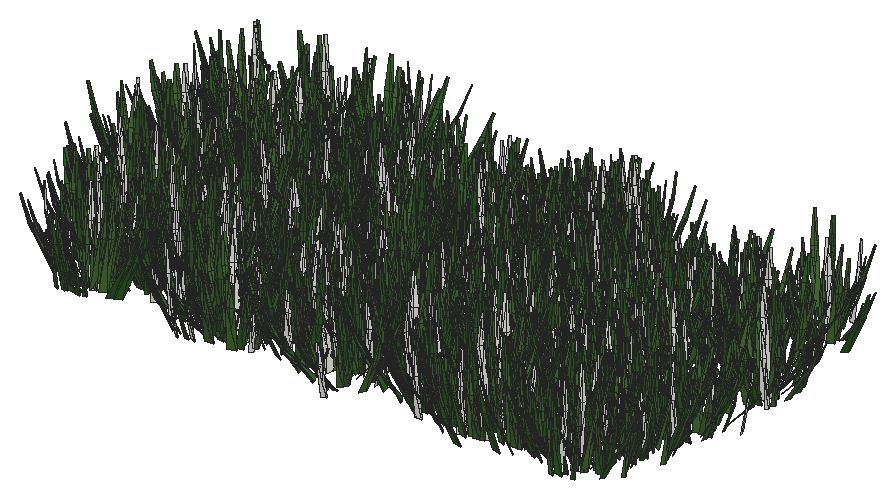
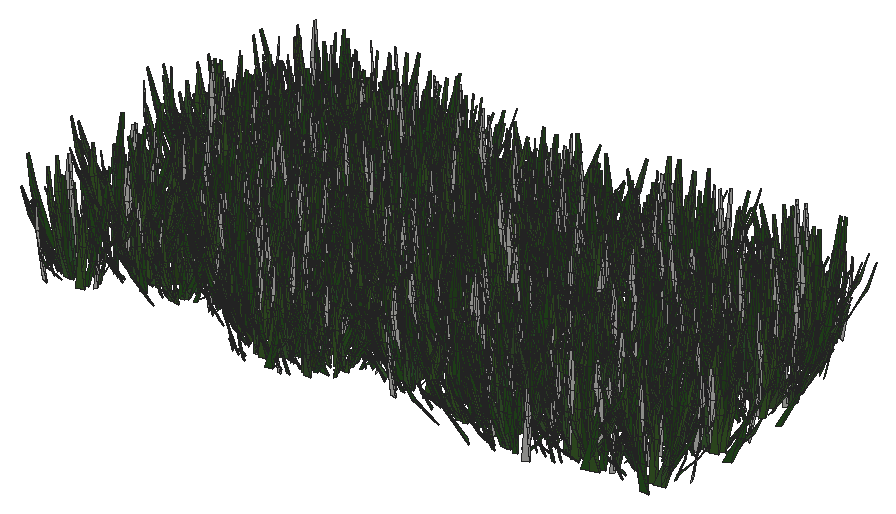
# SketchUp Ruby script. Lengths in inches.
U = 1.inch
M = Sketchup.active_model
def pt(a) = Geom::Point3d.new(a.map { |v| v * U })
def face(e, loops, mat)
  f = e.add_face(loops[0].map { |a| pt(a) })
  loops[1..].each { |l| e.add_face(l.map { |a| pt(a) }).erase! }
  f.material = f.back_material = mat if mat
  f
end
# faces: each face lists its corners as indices into pts; further lists are holes
def faces(e, pts, list, mat = nil) = list.each { |f| face(e, (f[0].is_a?(Array) ? f : [f]).map { |l| l.map { |i| pts[i] } }, mat) }
# xy, xz, yz: faces in a plane at the given z, y or x. An outline is a flat list of corners, or four numbers for a rectangle; further outlines are holes
def ring(l) = l.size == 4 ? [[l[0], l[1]], [l[2], l[1]], [l[2], l[3]], [l[0], l[3]]] : l.each_slice(2).to_a
def flat(e, list, mat, &to3) = list.each { |f| face(e, (f[0].is_a?(Array) ? f : [f]).map { |l| ring(l).map { |u, v| to3.(u, v) } }, mat) }
def xy(e, z, list, mat = nil) = flat(e, list, mat) { |x, y| [x, y, z] }
def xz(e, y, list, mat = nil) = flat(e, list, mat) { |x, z| [x, y, z] }
def yz(e, x, list, mat = nil) = flat(e, list, mat) { |y, z| [x, y, z] }
def lines(e, pts, list) = list.each { |a, b| e.add_line(pt(pts[a]), pt(pts[b])) }
# prism: a flat outline (further loops are holes) pulled along v
def prism(e, loops, v, mat = nil)
  f = face(e, loops, mat); d = Geom::Vector3d.new(v.map { |x| x * U })
  f.pushpull(f.normal.samedirection?(d) ? d.length : -d.length)
end
def box(e, o, s, mat = nil) = prism(e, [[o, [o[0] + s[0], o[1], o[2]], [o[0] + s[0], o[1] + s[1], o[2]], [o[0], o[1] + s[1], o[2]]]], [0, 0, s[2]], mat)
def at(x, y, z, deg = 0) = Geom::Transformation.translation(pt([x, y, z])) * Geom::Transformation.rotation(ORIGIN, Z_AXIS, deg.degrees)
def axes(o, x, y, z) = Geom::Transformation.new([*x, 0, *y, 0, *z, 0, *pt(o).to_a, 1])
def part(name) = M.definitions.add(name)
# library, detail: a bought-in or finely detailed component or shape, given as its bounding box
def library(name, o, s) = part(name).tap { |d| box(d.entities, o, s) }
def detail(e, o, s) = box(e.add_group.entities, o, s)
def put(e, d, t, mat = nil) = e.add_instance(d, t).tap { |i| i.material = mat if mat }
def group(e, t, mat = nil) = e.add_group.tap { |g| g.transformation = t; g.material = mat if mat }.entities
root = M.entities
M.materials.add("Material1").color = [58, 110, 58]
M.materials.add("Material10").color = [48, 100, 38]
M.materials.add("Material3").color = [68, 110, 58]
M.materials.add("Material4").color = [48, 90, 38]
M.materials.add("Material5").color = [68, 110, 48]
M.materials.add("Material6").color = [48, 90, 48]
M.materials.add("Material8").color = [58, 90, 38]
M.materials.add("Material9").color = [68, 100, 58]
c1 = part("grass00")
p = [[-0.6875,0.15,0],[-0.56,0.08,5.52],[-0.04,0.03,2.76],[0.48,-0.02,0],[0.35,-0.02,5.52],[-0.1,-0.14,5.52],
  [-0.12,0.65,8.37],[-0.42,0.65,8.37]]
faces(c1.entities,p,[[0,1,2,3],[3,2,4],[1,5,2],[5,4,2],[1,6,5],[4,5,6],[7,6,1]])
c2 = part("Group16\#1")
put(c2.entities,c1,axes([1.44,-0.61,-0.01],[0.05352,0.12609,0],[-0.10704,0.04543,0.07239],[0.06664,-0.02828,0.11628]),"Material6")
put(c2.entities,c1,axes([0.76,-0.15,-0.01],[0.04676,0.24062,0],[-0.23162,0.04501,0.06642],[0.0652,-0.01267,0.23595]),"Material3")
put(c2.entities,c1,axes([0.79,0.01,-0.01],[-0.00606,0.34651,0],[-0.34381,-0.00602,0.0432],[0.04319,0.00076,0.34386]))
put(c2.entities,c1,axes([1,0.23,-0.01],[-0.07192,0.31144,0],[-0.28722,-0.06632,0.1236],[0.12043,0.02781,0.29478]),"Material5")
put(c2.entities,c1,axes([1.66,0.77,-0.01],[-0.13828,0.29651,0],[-0.21551,-0.1005,0.22471],[0.20365,0.09498,0.23779]),"Material10")
put(c2.entities,c1,axes([0.6875,0.52,-0.01],[-0.18126,0.24051,0],[-0.22746,-0.17142,0.09788],[0.07817,0.05891,0.28481]),"Material5")
put(c2.entities,c1,axes([0.68,0.78,-0.01],[-0.215,0.18688,0],[-0.12385,-0.14248,0.21334],[0.13995,0.16101,0.18878]),"Material3")
put(c2.entities,c1,axes([0.56,1,-0.01],[-0.13756,0.07624,0],[-0.06159,-0.11112,0.0927],[0.04494,0.08108,0.12705]),"Material5")
put(c2.entities,c1,axes([0.2,0.64,-0.01],[-0.23729,0.07254,0],[-0.05711,-0.18681,0.153],[0.04473,0.14632,0.19535]),"Material10")
put(c2.entities,c1,axes([0.0625,0.72,-0.01],[-0.28874,0.02525,0],[-0.02179,-0.24916,0.14647],[0.01276,0.14591,0.25012]),"Material3")
put(c2.entities,c1,axes([-0.08,0.62,-0.01],[-0.34089,-0.04187,0],[0.03255,-0.26504,0.216],[-0.02633,0.21439,0.26703]),"Material10")
put(c2.entities,c1,axes([-0.34,0.98,-0.01],[-0.14314,-0.0493,0],[0.04397,-0.12769,0.06843],[-0.02228,0.0647,0.13505]),"Material10")
put(c2.entities,c1,axes([-0.87,1.45,-0.01],[-0.23488,-0.14114,0],[0.13761,-0.22901,0.06087],[-0.03135,0.05217,0.26717]))
put(c2.entities,c1,axes([-0.72,0.77,-0.01],[-0.14208,-0.13251,0],[0.07209,-0.0773,0.16301],[-0.11118,0.11922,0.1057]),"Material10")
put(c2.entities,c1,axes([-0.62,0.43,-0.01],[-0.14845,-0.21203,0],[0.18654,-0.13061,0.12304],[-0.10079,0.07057,0.22772]),"Material3")
put(c2.entities,c1,axes([-0.68,0.29,-0.01],[-0.13639,-0.32136,0],[0.31723,-0.13464,0.05579],[-0.05136,0.0218,0.34462]),"Material4")
put(c2.entities,c1,axes([-0.64,0.125,-0.01],[-0.0458,-0.23569,0],[0.22124,-0.043,0.08276],[-0.08124,0.01579,0.22538]),"Material1")
put(c2.entities,c1,axes([-1.6,-0.03,-0.01],[0.00576,-0.32897,0],[0.27526,0.00482,0.18018],[-0.18015,-0.00315,0.2753]),"Material5")
put(c2.entities,c1,axes([-1.36,-0.31,-0.01],[0.05718,-0.24765,0],[0.18172,0.04196,0.17267],[-0.16825,-0.03885,0.1865]),"Material10")
put(c2.entities,c1,axes([-1.54,-0.72,-0.01],[0.06537,-0.14017,0],[0.13555,0.06321,0.03939],[-0.0357,-0.01665,0.14956]))
put(c2.entities,c1,axes([-1.19,-0.9,-0.01],[0.09597,-0.12735,0],[0.11214,0.08451,0.07557],[-0.06035,-0.04548,0.14042]),"Material9")
put(c2.entities,c1,axes([-0.47,-0.54,-0.01],[0.11588,-0.10072,0],[0.0618,0.0711,0.12124],[-0.07953,-0.0915,0.0942]))
put(c2.entities,c1,axes([-0.47,-0.84,-0.01],[0.11927,-0.0661,0],[0.06603,0.11913,0.00646],[-0.00313,-0.00565,0.13621]),"Material5")
put(c2.entities,c1,axes([-0.38,-1.24,-0.01],[0.28037,-0.08571,0],[0.0618,0.20215,0.20315],[-0.05939,-0.19428,0.21139]),"Material9")
put(c2.entities,c1,axes([-0.06,-0.66,-0.01],[0.22719,-0.01987,0],[0.01247,0.14255,0.17758],[-0.01547,-0.17691,0.1431]),"Material8")
put(c2.entities,c1,axes([0.11,-0.89,-0.01],[0.14882,0.01828,0],[-0.01058,0.08611,0.12229],[0.01491,-0.12138,0.08676]),"Material6")
put(c2.entities,c1,axes([0.25,-0.72,-0.01],[0.20481,0.07053,0],[-0.06206,0.18022,0.10291],[0.03351,-0.0973,0.1906]),"Material6")
put(c2.entities,c1,axes([0.85,-1.42,-0.01],[0.16481,0.09904,0],[-0.09472,0.15762,0.05616],[0.02893,-0.04814,0.18389]),"Material5")
put(c2.entities,c1,axes([1.01,-1.09,-0.01],[0.21858,0.20385,0],[-0.17495,0.1876,0.15339],[0.10462,-0.11218,0.25652]),"Material10")
put(c2.entities,c1,axes([1.01,-0.71,-0.01],[0.08733,0.12473,0],[-0.06445,0.04512,0.13037],[0.1068,-0.07477,0.07867]),"Material6")
c3 = part("Group15\#1")
put(c3.entities,c2,at(0,0,0))
c4 = part("3darcstudiotree_grass00\#1")
put(c4.entities,c3,at(0,0,0))
put(root,c4,axes([299.78,141.87,0.25],[-0.51577,0.72337,0],[-1.03322,-0.50751,-0.04665],[-0.04944,-0.02429,1.47851]))
put(root,c4,axes([300.08,145.62,0.25],[0.04993,0.88338,0],[-1.12828,0.04393,-0.04808],[-0.07252,0.00282,1.70557]))
put(root,c4,axes([300.54,138.19,0.25],[-1.00125,0.60358,0],[-0.57545,-0.65762,-0.02785],[-0.03086,-0.03527,1.84622]))
put(root,c4,axes([300.73,137.15,0.25],[-0.28415,-0.883,0],[1.03818,-0.23015,-0.04991],[0.05947,-0.01318,1.32514]))
put(root,c4,axes([300.77,136.11,0.25],[0.54173,-0.92093,0],[0.98628,0.39968,-0.03421],[0.05303,0.02149,1.89316]))
put(root,c4,axes([301.14,134.74,0.25],[-0.01613,-0.76479,0],[1.13568,-0.0165,-0.04239],[0.05311,-0.00077,1.42343]))
put(root,c4,axes([301.49,140.1,0.25],[-0.02649,0.7502,0],[-0.93326,-0.0227,-0.04664],[-0.07074,-0.00172,1.41669]))
put(root,c4,axes([301.48,142.71,0.25],[0.76423,0.72762,0],[-0.68872,0.49833,-0.0286],[-0.04274,0.03093,1.81122]))
put(root,c4,axes([302.39,132.09,0.25],[-0.43129,0.73346,0],[-1.07574,-0.43577,-0.02753],[-0.03805,-0.01541,1.84121]))
put(root,c4,axes([302.49,133.8,0.25],[0.56343,-0.63153,0],[0.788,0.48432,-0.04843],[0.0685,0.0421,1.72564]))
put(root,c4,axes([303.03,137.14,0.25],[0.05508,-0.79039,0],[1.0526,0.05053,-0.03098],[0.04607,0.00221,1.57088]))
put(root,c4,axes([303.125,136.4375,0.25],[-0.10182,-0.84072,0],[1.03842,-0.08664,-0.02999],[0.05463,-0.00456,1.91089]))
put(root,c4,axes([303.05,145.8,0.25],[0.5504,-0.80783,0],[1.00535,0.47188,-0.04614],[0.05165,0.02424,1.48544]))
put(root,c4,axes([303.06,130.6,0.25],[0.88072,-0.75596,0],[0.79178,0.63548,-0.03201],[0.03942,0.03164,1.88682]))
put(root,c4,axes([303.72,130.48,0.25],[0.67514,-0.58996,0],[0.84636,0.66723,-0.03691],[0.04374,0.03448,1.90749]))
put(root,c4,axes([304.05,135.15,0.25],[-0.82491,-0.8058,0],[0.91289,-0.64381,-0.06095],[0.06828,-0.04816,1.76096]))
put(root,c4,axes([304.2,140.98,0.25],[-1.06648,-0.29234,0],[0.33481,-0.84142,-0.04962],[0.02631,-0.06612,1.8049]))
put(root,c4,axes([304.03,136.32,0.25],[-0.77838,0.37748,0],[-0.59922,-0.85123,-0.05376],[-0.03154,-0.04481,1.38154]))
put(root,c4,axes([303.89,142.53,0.25],[-0.25153,0.98585,0],[-1.19968,-0.21086,-0.05285],[-0.07259,-0.01276,1.72177]))
put(root,c4,axes([304.6,139.4,0.25],[-1.0477,-0.13596,0],[0.1947,-1.03362,-0.04342],[0.00888,-0.04717,1.66984]))
put(root,c4,axes([304.31,145.87,0.25],[-0.53647,0.96882,0],[-1.0534,-0.40184,-0.02861],[-0.04227,-0.01613,1.88512]))
put(root,c4,axes([304.62,138.11,0.25],[-0.94495,-0.04978,0],[0.07876,-1.02991,-0.04372],[0.00292,-0.03822,1.31241]))
put(root,c4,axes([304.66,133.875,0.25],[0.88611,-0.32919,0],[0.4327,0.80239,-0.04939],[0.03441,0.06381,1.80606]))
put(root,c4,axes([305.41,132.12,0.25],[-0.97721,-0.2509,0],[0.37297,-1.00075,-0.06046],[0.02106,-0.05652,1.48798]))
put(root,c4,axes([306.02,142.74,0.25],[1.14716,0.41931,0],[-0.39995,0.75378,-0.04159],[-0.02402,0.04527,1.42181]))
put(root,c4,axes([306.17,139.4375,0.25],[0.27344,1.00751,0],[-1.06134,0.19844,-0.04632],[-0.06652,0.01244,1.6013]))
put(root,c4,axes([307.21,143.59,0.25],[-0.92535,-0.73173,0],[0.88977,-0.77516,-0.03405],[0.02665,-0.02322,1.46358]))
put(root,c4,axes([306.67,138.9,0.25],[0.38479,0.87258,0],[-1.09891,0.33384,-0.03042],[-0.03924,0.01192,1.60735]))
put(root,c4,axes([306.79,147.18,0.25],[1.0966,0.3645,0],[-0.41445,0.85898,-0.05201],[-0.03051,0.06323,1.75905]))
put(root,c4,axes([307.11,134.75,0.25],[-0.02724,0.8884,0],[-1.06639,-0.02253,-0.03168],[-0.04928,-0.00104,1.66016]))
put(root,c4,axes([307.14,142.44,0.25],[0.47063,0.99955,0],[-1.01276,0.3285,-0.05423],[-0.06364,0.02064,1.37014]))
put(root,c4,axes([307.41,133.73,0.25],[-0.66435,0.90789,0],[-1.02818,-0.5183,-0.06137],[-0.06369,-0.03211,1.46064]))
put(root,c4,axes([307.32,136.98,0.25],[0.98353,-0.2674,0],[0.31916,0.80872,-0.03684],[0.0181,0.04586,1.61813]))
put(root,c4,axes([307.6,145.88,0.25],[0.72927,0.8559,0],[-0.97666,0.57329,-0.03132],[-0.03828,0.02247,1.7905]))
put(root,c4,axes([308.45,141.2,0.25],[-0.57612,-0.75798,0],[0.99797,-0.52255,-0.04882],[0.04842,-0.02535,1.38366]))
put(root,c4,axes([308.22,138.1,0.25],[1.07822,-0.4599,0],[0.58685,0.94782,-0.04443],[0.02209,0.03568,1.39643]))
put(root,c4,axes([308.5625,143.11,0.25],[-0.5579,-0.63099,0],[1.01432,-0.61782,-0.05528],[0.06314,-0.03846,1.78248]))
put(root,c4,axes([308.57,142.55,0.25],[-1.00665,-0.38225,0],[0.39719,-0.72058,-0.02741],[0.0223,-0.04045,1.86713]))
put(root,c4,axes([308.5625,131.11,0.25],[-0.96516,0.38443,0],[-0.43122,-0.74583,-0.02803],[-0.02343,-0.04053,1.92571]))
put(root,c4,axes([308.45,139.83,0.25],[1.05725,-0.32469,0],[0.33364,0.74841,-0.04569],[0.02936,0.06585,1.78027]))
put(root,c4,axes([308.57,133.29,0.25],[1.21894,-0.05836,0],[0.05945,0.85542,-0.03809],[0.00382,0.05491,1.79573]))
put(root,c4,axes([308.69,132.48,0.25],[1.08674,-0.51423,0],[0.5096,0.74191,-0.05304],[0.04758,0.06927,1.86337]))
put(root,c4,axes([309.62,144.6875,0.25],[0.96211,-0.31155,0],[0.3285,0.69886,-0.03886],[0.02375,0.05053,1.52001]))
put(root,c4,axes([309.84,133.23,0.25],[0.18176,0.81903,0],[-1.09456,0.16733,-0.0472],[-0.06112,0.00934,1.46547]))
put(root,c4,axes([309.86,146.21,0.25],[0.71429,0.86085,0],[-0.78996,0.45156,-0.04649],[-0.05198,0.02971,1.30192]))
put(root,c4,axes([309.89,139.42,0.25],[1.04874,0.16215,0],[-0.17266,0.76932,-0.03922],[-0.01113,0.04958,1.46066]))
put(root,c4,axes([310.47,137,0.25],[-0.34398,-0.78173,0],[0.86639,-0.26263,-0.03784],[0.06395,-0.01938,1.65933]))
put(root,c4,axes([310.63,141.27,0.25],[1.04153,-0.54846,0],[0.60752,0.79477,-0.04672],[0.04077,0.05334,1.84728]))
put(root,c4,axes([310.46,130.5625,0.25],[0.92621,0.73809,0],[-0.85701,0.74087,-0.04664],[-0.04646,0.04016,1.77978]))
put(root,c4,axes([311.28,143.21,0.25],[0.57087,-0.64299,0],[0.86179,0.52709,-0.04551],[0.05625,0.0344,1.64335]))
put(root,c4,axes([311.53,130.5625,0.25],[-0.46204,0.65988,0],[-1.12301,-0.5417,-0.02835],[-0.03266,-0.01575,1.73088]))
put(root,c4,axes([312.01,144.46,0.25],[-1.01342,0.10573,0],[-0.15227,-1.00541,-0.04842],[-0.00964,-0.06363,1.94818]))
put(root,c4,axes([311.79,142.55,0.25],[1.26054,0.10801,0],[-0.1304,1.04837,-0.06196],[-0.00771,0.06201,1.53928]))
put(root,c4,axes([311.85,134.45,0.25],[1.00305,0.14539,0],[-0.20705,0.98408,-0.04039],[-0.00807,0.03835,1.39779]))
put(root,c4,axes([311.91,141.29,0.25],[0.92598,0.55829,0],[-0.67255,0.76846,-0.05492],[-0.04623,0.05283,1.63919]))
put(root,c4,axes([312.95,132.18,0.25],[-1.15018,-0.15887,0],[0.16599,-0.8279,-0.03971],[0.00952,-0.04747,1.4765]))
put(root,c4,axes([312.78,136.05,0.25],[0.82997,-0.75391,0],[0.73924,0.56064,-0.04297],[0.04689,0.03556,1.48019]))
put(root,c4,axes([313.24,141.47,0.25],[0.34968,-0.96719,0],[0.98733,0.24591,-0.0465],[0.06293,0.01567,1.45674]))
put(root,c4,axes([312.98,134.48,0.25],[1.12096,-0.03668,0],[0.04224,0.88921,-0.03451],[0.00237,0.04996,1.8714]))
put(root,c4,axes([312.97,133.34,0.25],[0.94146,0.27887,0],[-0.40298,0.93723,-0.03925],[-0.0143,0.03327,1.29995]))
put(root,c4,axes([313.625,139.54,0.25],[-0.01858,-0.90757,0],[1.28861,-0.01817,-0.0635],[0.09505,-0.00134,1.92948]))
put(root,c4,axes([313.75,145.91,0.25],[0.98461,-0.38374,0],[0.39191,0.69275,-0.03796],[0.02677,0.04732,1.52986]))
put(root,c4,axes([314.42,143.93,0.25],[-0.34623,-0.72321,0],[1.04472,-0.34455,-0.04918],[0.05465,-0.01802,1.34418]))
put(root,c4,axes([314.54,145.03,0.25],[0.15043,-0.7527,0],[1.21044,0.16665,-0.06063],[0.07503,0.01033,1.53907]))
put(root,c4,axes([314.73,138.17,0.25],[0.39909,-0.81566,0],[1.02034,0.34393,-0.04502],[0.07048,0.02376,1.86083]))
put(root,c4,axes([314.98,133.11,0.25],[-0.27504,-0.89282,0],[1.07963,-0.22912,-0.04783],[0.06688,-0.01419,1.6084]))
put(root,c4,axes([314.77,131.41,0.25],[1.24297,0.07238,0],[-0.08345,0.98727,-0.05051],[-0.00566,0.06702,1.91076]))
put(root,c4,axes([315.16,136.78,0.25],[0.44545,-0.68346,0],[1.06425,0.47785,-0.03985],[0.0435,0.01953,1.5017]))
put(root,c4,axes([315.03,142.12,0.25],[1.14321,0.40608,0],[-0.51013,0.98935,-0.06274],[-0.03659,0.07096,1.92197]))
put(root,c4,axes([315.69,137.68,0.25],[-1.0413,-0.45924,0],[0.51605,-0.8061,-0.03648],[0.0279,-0.04359,1.79293]))
put(root,c4,axes([316.17,132.56,0.25],[0.8304,0.29143,0],[-0.37726,0.74054,-0.04149],[-0.03179,0.0624,1.90578]))
put(root,c4,axes([316.15,133.21,0.25],[1.10631,0.33098,0],[-0.3979,0.91621,-0.05978],[-0.02583,0.05947,1.49495]))
put(root,c4,axes([316.4375,134.86,0.25],[0.42473,-0.75301,0],[0.8196,0.31847,-0.04141],[0.08184,0.0318,1.97468]))
put(root,c4,axes([316.54,141.47,0.25],[-0.21123,0.7691,0],[-0.89914,-0.17012,-0.03421],[-0.06786,-0.01284,1.87625]))
put(root,c4,axes([317.21,133.19,0.25],[-1.12613,-0.03411,0],[0.04109,-0.93447,-0.04384],[0.00237,-0.05387,1.66887]))
put(root,c4,axes([317.4375,131.97,0.25],[-0.97309,0.51402,0],[-0.49262,-0.64245,-0.04609],[-0.04607,-0.06009,1.7083]))
put(root,c4,axes([317.63,134.71,0.25],[-0.64125,-0.58627,0],[0.90023,-0.67833,-0.05879],[0.05947,-0.04481,1.66118]))
put(root,c4,axes([317.62,130.52,0.25],[-0.97091,0.18786,0],[-0.29032,-1.03362,-0.06463],[-0.01526,-0.05435,1.33032]))
put(root,c4,axes([317.6875,142.18,0.25],[-0.0786,-0.93173,0],[1.13363,-0.06588,-0.04142],[0.06279,-0.00365,1.72685]))
put(root,c4,axes([317.33,146.08,0.25],[0.35004,0.7486,0],[-1.10063,0.35454,-0.04732],[-0.05301,0.01708,1.41896]))
put(root,c4,axes([317.71,140.87,0.25],[1.16212,0.12281,0],[-0.11865,0.77346,-0.04636],[-0.01154,0.07525,1.85211]))
put(root,c4,axes([318.25,147.34,0.25],[-0.69384,-0.6726,0],[0.85793,-0.60969,-0.03189],[0.03287,-0.02336,1.53238]))
put(root,c4,axes([318.26,138.55,0.25],[0.89894,0.06975,0],[-0.1065,0.94557,-0.04931],[-0.00617,0.05478,1.538]))
put(root,c4,axes([318.9,142.34,0.25],[0.3076,0.88313,0],[-0.9496,0.22786,-0.04889],[-0.06973,0.01673,1.46761]))
put(root,c4,axes([319.32,133.625,0.25],[0.44989,-0.65828,0],[1.12235,0.52842,-0.03953],[0.04723,0.02224,1.77239]))
put(root,c4,axes([319.52,138.32,0.25],[-0.95818,-0.32844,0],[0.39605,-0.79597,-0.04671],[0.03185,-0.06401,1.85324]))
put(root,c4,axes([319.27,134.52,0.25],[0.25037,1.00901,0],[-1.01055,0.17274,-0.03105],[-0.05539,0.00947,1.87912]))
put(root,c4,axes([319.34,137.24,0.25],[0.35055,1.00246,0],[-0.90433,0.21786,-0.03743],[-0.0536,0.01291,1.40382]))
put(root,c4,axes([319.48,143.4,0.25],[0.66113,0.53342,0],[-0.84049,0.71763,-0.04673],[-0.03929,0.03355,1.45453]))
put(root,c4,axes([319.6,144.55,0.25],[1.17347,-0.27786,0],[0.3552,1.03341,-0.04256],[0.01402,0.0408,1.55488]))
put(root,c4,axes([319.69,145.62,0.25],[0.1752,0.94217,0],[-0.95925,0.12288,-0.04631],[-0.07803,0.01,1.65491]))
put(root,c4,axes([319.8125,146.87,0.25],[0.28963,0.74847,0],[-0.93547,0.24938,-0.04361],[-0.06802,0.01813,1.60948]))
put(root,c4,axes([320.26,139.86,0.25],[-0.06585,-0.80008,0],[1.09119,-0.06187,-0.04502],[0.05343,-0.00303,1.30109]))
put(root,c4,axes([320.76,147.34,0.25],[-0.46015,0.96018,0],[-0.861,-0.28426,-0.04072],[-0.06272,-0.02071,1.53595]))
put(root,c4,axes([320.88,141.8,0.25],[1.02393,-0.20893,0],[0.23736,0.80136,-0.02888],[0.01203,0.04061,1.73467]))
put(root,c4,axes([321.84,131.28,0.25],[-1.12621,0.19113,0],[-0.2015,-0.81791,-0.0347],[-0.01115,-0.04525,1.61275]))
put(root,c4,axes([322.08,140.71,0.25],[0.06137,-0.83271,0],[1.13269,0.05751,-0.05271],[0.06386,0.00324,1.37729]))
put(root,c4,axes([322.02,131.74,0.25],[0.54931,-0.6716,0],[0.75634,0.42617,-0.03969],[0.0509,0.02868,1.41714]))
put(root,c4,axes([322.27,138.85,0.25],[-0.78066,-0.67204,0],[0.68687,-0.54967,-0.03577],[0.04031,-0.03226,1.49339]))
put(root,c4,axes([321.93,137.24,0.25],[0.27982,0.75631,0],[-1.1229,0.28621,-0.03259],[-0.04697,0.01197,1.77089]))
put(root,c4,axes([321.93,145.23,0.25],[0.80316,0.707,0],[-0.70311,0.55026,-0.02839],[-0.0403,0.03154,1.88589]))
put(root,c4,axes([322.77,145.93,0.25],[-1.10827,0.13604,0],[-0.16547,-0.92861,-0.04443],[-0.01051,-0.05896,1.82802]))
put(root,c4,axes([323.32,142.65,0.25],[-0.86841,-0.52371,0],[0.68358,-0.78087,-0.03763],[0.03701,-0.04227,1.94544]))
put(root,c4,axes([323.41,137.35,0.25],[-0.91874,-0.68883,0],[0.79509,-0.73056,-0.0585],[0.0631,-0.05798,1.90866]))
put(root,c4,axes([323.25,141.46,0.25],[-0.34506,0.75478,0],[-0.92362,-0.29088,-0.03389],[-0.05306,-0.01671,1.65454]))
put(root,c4,axes([323.57,131.22,0.25],[-0.92977,-0.22168,0],[0.33206,-0.95946,-0.05258],[0.02224,-0.06426,1.84274]))
put(root,c4,axes([323.69,135.52,0.25],[-0.02074,-0.84875,0],[1.20005,-0.0202,-0.05384],[0.05935,-0.001,1.32332]))
put(root,c4,axes([323.71,145.12,0.25],[-1.03502,0.33572,0],[-0.32811,-0.69686,-0.02866],[-0.02179,-0.04627,1.88291]))
put(root,c4,axes([323.92,140.11,0.25],[-0.92041,-0.50708,0],[0.71428,-0.89316,-0.03911],[0.02409,-0.03012,1.43856]))
put(root,c4,axes([323.76,134.42,0.25],[-0.00089,-0.79123,0],[0.93063,-0.00072,-0.0371],[0.07359,-0.00006,1.84609]))
put(root,c4,axes([323.72,133.85,0.25],[0.98992,-0.58841,0],[0.73097,0.84717,-0.04389],[0.03917,0.04539,1.92393]))
put(root,c4,axes([324.01,132.55,0.25],[1.03159,-0.24301,0],[0.31461,0.92006,-0.03157],[0.01327,0.0388,1.77323]))
put(root,c4,axes([324.93,137.42,0.25],[-0.37538,-0.75879,0],[1.02359,-0.34885,-0.04381],[0.0639,-0.02178,1.74465]))
put(root,c4,axes([325.22,130.91,0.25],[-0.31286,-1.00069,0],[0.95551,-0.2058,-0.03225],[0.05006,-0.01078,1.58326]))
put(root,c4,axes([325.21,139.4,0.25],[-0.68886,0.65962,0],[-0.76509,-0.55044,-0.04719],[-0.04586,-0.033,1.30223]))
put(root,c4,axes([325.4375,132.06,0.25],[-1.1496,0.19764,0],[-0.26311,-1.05431,-0.05761],[-0.01547,-0.06199,1.71741]))
put(root,c4,axes([325.21,143.875,0.25],[0.88062,-0.61517,0],[0.61619,0.60767,-0.04982],[0.04793,0.04726,1.4295]))
put(root,c4,axes([325.77,140.73,0.25],[-1.01365,-0.2867,0],[0.41301,-1.00597,-0.06303],[0.02557,-0.06229,1.61067]))
put(root,c4,axes([325.49,135.15,0.25],[-0.09408,0.90156,0],[-0.94702,-0.06808,-0.04948],[-0.07382,-0.00531,1.42361]))
put(root,c4,axes([325.37,138.35,0.25],[0.48298,0.67524,0],[-0.96114,0.47361,-0.05173],[-0.05494,0.02707,1.38038]))
put(root,c4,axes([325.57,136.02,0.25],[1.24776,-0.01262,0],[0.01151,0.78391,-0.04731],[0.00097,0.06603,1.58849]))
put(root,c4,axes([326.68,142.55,0.25],[-1.07098,0.00098,0],[-0.0011,-0.82988,-0.04481],[-0.00008,-0.06336,1.70362]))
put(root,c4,axes([326.99,131.33,0.25],[-0.38232,-0.8248,0],[1.0254,-0.32744,-0.0371],[0.06184,-0.01975,1.96201]))
put(root,c4,axes([326.6875,145.81,0.25],[0.61629,0.74541,0],[-0.84229,0.47975,-0.0512],[-0.05744,0.03271,1.38975]))
put(root,c4,axes([326.875,141,0.25],[-0.48948,0.79426,0],[-0.95032,-0.40345,-0.05082],[-0.05731,-0.02433,1.35221]))
put(root,c4,axes([326.68,140.01,0.25],[0.87338,0.77655,0],[-0.84307,0.65321,-0.04297],[-0.054,0.04184,1.98261]))
put(root,c4,axes([327.08,143.14,0.25],[-0.95799,0.61503,0],[-0.71197,-0.76397,-0.05181],[-0.03955,-0.04244,1.45196]))
put(root,c4,axes([327.14,138.92,0.25],[-1.01325,0.457,0],[-0.60843,-0.92932,-0.04664],[-0.02856,-0.04362,1.63424]))
put(root,c4,axes([327.33,136.96,0.25],[0.76856,-0.67545,0],[0.83236,0.65245,-0.05261],[0.04639,0.03636,1.38839]))
put(root,c4,axes([327.87,136.03,0.25],[-0.22788,-0.74237,0],[0.90783,-0.19197,-0.03395],[0.05396,-0.01141,1.53644]))
put(root,c4,axes([327.96,138.12,0.25],[-0.11967,-0.81693,0],[1.27003,-0.12816,-0.04217],[0.04627,-0.00467,1.41426]))
put(root,c4,axes([327.81,141.34,0.25],[1.06326,-0.22826,0],[0.31162,0.99997,-0.04841],[0.01731,0.05555,1.77682]))
put(root,c4,axes([328.2,132.15,0.25],[-0.23429,-0.89921,0],[1.23928,-0.22244,-0.05631],[0.0599,-0.01075,1.37991]))
put(root,c4,axes([328.5,131.36,0.25],[-0.77366,-0.45207,0],[0.59884,-0.70602,-0.03828],[0.04199,-0.0495,1.98208]))
put(root,c4,axes([328.51,136.89,0.25],[1.09162,0.12033,0],[-0.16865,1.054,-0.05242],[-0.01009,0.06305,1.87281]))
put(root,c4,axes([328.79,145.66,0.25],[-0.08305,0.76668,0],[-0.93277,-0.0696,-0.0349],[-0.0526,-0.00392,1.41691]))
put(root,c4,axes([329.68,132.47,0.25],[-0.76849,-0.52302,0],[0.63142,-0.63915,-0.04795],[0.04245,-0.04297,1.39039]))
put(root,c4,axes([329.74,143.0625,0.25],[-0.39413,-0.9358,0],[1.01758,-0.29524,-0.03865],[0.0656,-0.01903,1.9383]))
put(root,c4,axes([330.125,136.41,0.25],[-0.85575,-0.43191,0],[0.66605,-0.9091,-0.06276],[0.03807,-0.05197,1.49667]))
put(root,c4,axes([329.68,133.7,0.25],[0.81477,0.44609,0],[-0.56799,0.71467,-0.03997],[-0.03926,0.0494,1.84008]))
put(root,c4,axes([330.02,136.82,0.25],[-0.18041,0.88952,0],[-1.05657,-0.14763,-0.04712],[-0.05773,-0.00807,1.33133]))
put(root,c4,axes([330.26,130.97,0.25],[0.9962,-0.46147,0],[0.50997,0.75841,-0.03495],[0.03097,0.04605,1.90256]))
put(root,c4,axes([330.82,137.3125,0.25],[-0.30521,0.9712,0],[-1.05653,-0.22873,-0.04083],[-0.06972,-0.01509,1.92702]))
put(root,c4,axes([331.2,144.68,0.25],[-0.90516,0.46904,0],[-0.66226,-0.88044,-0.02972],[-0.02044,-0.02717,1.62371]))
put(root,c4,axes([331.625,134.89,0.25],[-0.99885,-0.03422,0],[0.05154,-1.03638,-0.05407],[0.00301,-0.06042,1.68402]))
put(root,c4,axes([331.23,131.95,0.25],[0.64903,0.54556,0],[-0.89812,0.73605,-0.04002],[-0.04121,0.03377,1.82631]))
put(root,c4,axes([331.79,136.04,0.25],[-1.20408,-0.1285,0],[0.12563,-0.81098,-0.03967],[0.00916,-0.05911,1.78282]))
put(root,c4,axes([331.61,147.21,0.25],[0.81525,-0.75674,0],[0.80305,0.596,-0.03435],[0.04365,0.0324,1.83666]))
put(root,c4,axes([331.88,133.53,0.25],[0.79979,0.77322,0],[-0.80748,0.57539,-0.03135],[-0.03902,0.0278,1.74596]))
put(root,c4,axes([332.36,142.08,0.25],[-1.19693,-0.05294,0],[0.06044,-0.94137,-0.04256],[0.00333,-0.05193,1.67228]))
put(root,c4,axes([332.54,137.33,0.25],[-0.17919,-0.94615,0],[1.2585,-0.16419,-0.0381],[0.05711,-0.00745,1.93318]))
put(root,c4,axes([332.81,141.29,0.25],[-0.30663,0.87951,0],[-1.19559,-0.28715,-0.06381],[-0.0822,-0.01974,1.66913]))
